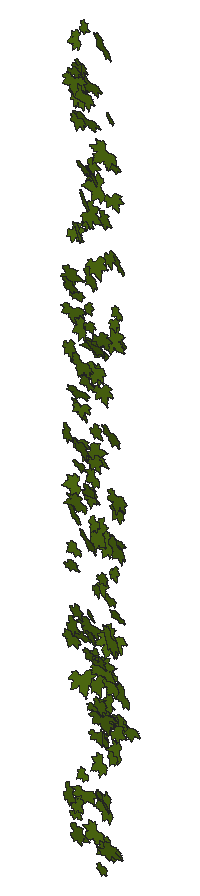
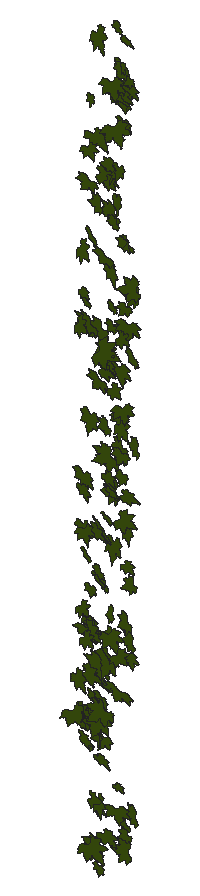
# SketchUp Ruby script. Lengths in inches.
U = 1.inch
M = Sketchup.active_model
def pt(a) = Geom::Point3d.new(a.map { |v| v * U })
def face(e, loops, mat)
  f = e.add_face(loops[0].map { |a| pt(a) })
  loops[1..].each { |l| e.add_face(l.map { |a| pt(a) }).erase! }
  f.material = f.back_material = mat if mat
  f
end
# faces: each face lists its corners as indices into pts; further lists are holes
def faces(e, pts, list, mat = nil) = list.each { |f| face(e, (f[0].is_a?(Array) ? f : [f]).map { |l| l.map { |i| pts[i] } }, mat) }
# xy, xz, yz: faces in a plane at the given z, y or x. An outline is a flat list of corners, or four numbers for a rectangle; further outlines are holes
def ring(l) = l.size == 4 ? [[l[0], l[1]], [l[2], l[1]], [l[2], l[3]], [l[0], l[3]]] : l.each_slice(2).to_a
def flat(e, list, mat, &to3) = list.each { |f| face(e, (f[0].is_a?(Array) ? f : [f]).map { |l| ring(l).map { |u, v| to3.(u, v) } }, mat) }
def xy(e, z, list, mat = nil) = flat(e, list, mat) { |x, y| [x, y, z] }
def xz(e, y, list, mat = nil) = flat(e, list, mat) { |x, z| [x, y, z] }
def yz(e, x, list, mat = nil) = flat(e, list, mat) { |y, z| [x, y, z] }
def lines(e, pts, list) = list.each { |a, b| e.add_line(pt(pts[a]), pt(pts[b])) }
# prism: a flat outline (further loops are holes) pulled along v
def prism(e, loops, v, mat = nil)
  f = face(e, loops, mat); d = Geom::Vector3d.new(v.map { |x| x * U })
  f.pushpull(f.normal.samedirection?(d) ? d.length : -d.length)
end
def box(e, o, s, mat = nil) = prism(e, [[o, [o[0] + s[0], o[1], o[2]], [o[0] + s[0], o[1] + s[1], o[2]], [o[0], o[1] + s[1], o[2]]]], [0, 0, s[2]], mat)
def at(x, y, z, deg = 0) = Geom::Transformation.translation(pt([x, y, z])) * Geom::Transformation.rotation(ORIGIN, Z_AXIS, deg.degrees)
def axes(o, x, y, z) = Geom::Transformation.new([*x, 0, *y, 0, *z, 0, *pt(o).to_a, 1])
def part(name) = M.definitions.add(name)
# library, detail: a bought-in or finely detailed component or shape, given as its bounding box
def library(name, o, s) = part(name).tap { |d| box(d.entities, o, s) }
def detail(e, o, s) = box(e.add_group.entities, o, s)
def put(e, d, t, mat = nil) = e.add_instance(d, t).tap { |i| i.material = mat if mat }
def group(e, t, mat = nil) = e.add_group.tap { |g| g.transformation = t; g.material = mat if mat }.entities
root = M.entities
M.materials.add("[Vegetation Blur 03]").color = [83, 114, 18]
c1 = part("ivy")
xy(c1.entities,0,[[0.782,0,0.786,0,0.787,0.005,0.789,0.009,0.821,0.072,0.875,0.147,1.001,0.272,1.073,0.331,1.137,0.363,1.178,0.379,1.223,0.384,1.272,0.383,1.311,0.374,1.36,0.355,1.399,0.334,1.491,0.285,1.541,0.244,1.583,0.199,1.617,0.15,1.64,0.128,1.662,0.115,1.717,0.105,1.745,0.093,1.784,0.054,1.819,0.057,1.854,0.064,1.882,0.075,1.896,0.074,1.91,0.071,1.937,0.063,1.964,0.053,1.99,0.038,2.016,0.015,2.034,0.002,2.04,0,2.038,0.003,2.036,0.007,2.033,0.038,2.036,0.068,2.045,0.1,2.055,0.116,2.064,0.123,2.077,0.129,2.088,0.129,2.106,0.132,2.118,0.13,2.179,0.132,2.207,0.133,2.225,0.133,2.242,0.138,2.22,0.162,2.207,0.186,2.206,0.213,2.212,0.236,2.228,0.262,2.247,0.274,2.298,0.283,2.355,0.294,2.37,0.296,2.376,0.295,2.377,0.3,2.377,0.303,2.385,0.329,2.411,0.37,2.426,0.392,2.449,0.407,2.511,0.426,2.561,0.444,2.619,0.466,2.589,0.469,2.561,0.476,2.501,0.5,2.449,0.516,2.424,0.523,2.401,0.535,2.377,0.556,2.372,0.568,2.36,0.575,2.268,0.586,2.225,0.592,2.207,0.599,2.194,0.61,2.143,0.65,2.13,0.664,2.122,0.682,2.123,0.7,2.13,0.719,2.148,0.75,2.17,0.781,2.195,0.807,2.221,0.828,2.284,0.874,2.291,0.88,2.288,0.887,2.276,0.9,2.267,0.916,2.265,0.933,2.273,0.967,2.292,1.002,2.313,1.03,2.334,1.054,2.348,1.067,2.358,1.074,2.363,1.076,2.362,1.081,2.35,1.094,2.347,1.11,2.35,1.143,2.359,1.18,2.385,1.254,2.415,1.324,2.448,1.393,2.45,1.4,2.446,1.398,2.44,1.394,2.427,1.383,2.402,1.36,2.376,1.339,2.345,1.324,2.305,1.309,2.282,1.303,2.273,1.306,2.245,1.294,2.212,1.287,2.187,1.291,2.163,1.301,2.142,1.316,2.134,1.327,2.124,1.325,2.09,1.292,2.053,1.259,2.014,1.234,1.973,1.215,1.954,1.21,1.931,1.208,1.909,1.212,1.893,1.22,1.879,1.233,1.872,1.248,1.867,1.281,1.864,1.319,1.821,1.258,1.773,1.197,1.726,1.141,1.698,1.121,1.679,1.116,1.666,1.117,1.647,1.122,1.632,1.129,1.62,1.141,1.617,1.154,1.617,1.219,1.621,1.254,1.623,1.268,1.623,1.281,1.618,1.314,1.606,1.346,1.603,1.375,1.607,1.403,1.603,1.467,1.599,1.499,1.605,1.525,1.614,1.552,1.629,1.577,1.635,1.589,1.629,1.587,1.618,1.582,1.596,1.566,1.581,1.556,1.568,1.552,1.557,1.55,1.545,1.553,1.531,1.562,1.522,1.572,1.504,1.591,1.486,1.611,1.474,1.631,1.457,1.666,1.455,1.684,1.457,1.698,1.452,1.715,1.444,1.728,1.424,1.754,1.419,1.772,1.423,1.786,1.434,1.819,1.444,1.848,1.446,1.855,1.44,1.861,1.43,1.867,1.386,1.904,1.349,1.948,1.326,1.973,1.31,1.995,1.288,2.048,1.284,2.153,1.287,2.254,1.284,2.255,1.282,2.253,1.278,2.247,1.274,2.237,1.266,2.216,1.226,2.125,1.208,2.076,1.184,2.033,1.155,1.984,1.135,1.942,1.111,1.899,1.083,1.861,1.053,1.85,1.059,1.83,1.061,1.809,1.056,1.79,1.049,1.767,1.04,1.749,1.018,1.733,0.994,1.726,0.942,1.734,0.95,1.6875,0.944,1.645,0.932,1.608,0.911,1.585,0.881,1.58,0.854,1.582,0.828,1.588,0.785,1.618,0.773,1.625,0.775,1.614,0.779,1.598,0.796,1.502,0.818,1.402,0.861,1.283,0.882,1.224,0.894,1.174,0.892,1.148,0.886,1.123,0.881,1.107,0.872,1.099,0.849,1.094,0.818,1.092,0.789,1.098,0.762,1.107,0.753,1.113,0.721,1.139,0.698,1.163,0.678,1.194,0.665,1.224,0.628,1.28,0.612,1.312,0.606,1.327,0.606,1.314,0.599,1.282,0.594,1.267,0.581,1.256,0.544,1.245,0.512,1.244,0.473,1.249,0.444,1.256,0.382,1.288,0.339,1.306,0.324,1.316,0.317,1.324,0.309,1.326,0.27,1.314,0.227,1.313,0.185,1.3125,0.152,1.317,0.122,1.328,0.092,1.345,0.073,1.353,0.079,1.338,0.092,1.308,0.117,1.249,0.13,1.215,0.139,1.164,0.147,1.148,0.157,1.136,0.163,1.122,0.174,1.086,0.177,1.067,0.182,1.054,0.186,1.043,0.191,1.038,0.211,1.028,0.237,1.005,0.25,0.974,0.253,0.96,0.25,0.944,0.242,0.914,0.243,0.906,0.249,0.902,0.26,0.894,0.289,0.88,0.307,0.873,0.322,0.862,0.364,0.799,0.403,0.738,0.431,0.709,0.439,0.691,0.441,0.678,0.4375,0.66,0.428,0.645,0.394,0.623,0.303,0.594,0.255,0.581,0.214,0.577,0.179,0.573,0.173,0.568,0.175,0.561,0.167,0.55,0.141,0.523,0.113,0.503,0.077,0.49,0.045,0.486,0.026,0.485,0.019,0.486,0.011,0.483,0,0.471,0.014,0.467,0.044,0.455,0.058,0.447,0.07,0.438,0.097,0.411,0.125,0.394,0.158,0.377,0.174,0.366,0.182,0.359,0.185,0.361,0.242,0.331,0.253,0.316,0.258,0.303,0.262,0.283,0.274,0.278,0.308,0.274,0.341,0.252,0.366,0.226,0.366,0.222,0.37,0.22,0.38,0.221,0.395,0.221,0.425,0.216,0.45,0.207,0.465,0.192,0.473,0.178,0.484,0.15,0.489,0.116,0.483,0.089,0.468,0.058,0.45,0.035,0.435,0.018,0.429,0.011,0.434,0.012,0.438,0.014,0.469,0.019,0.542,0.016,0.581,0.015,0.612,0.027,0.68,0.055,0.696,0.057,0.712,0.052,0.73,0.045,0.741,0.036,0.766,0.014]])
put(root,c1,axes([125.75,173.7,113.6875],[0.43906,-0.08807,-0.12908],[-0.15747,0.03053,-0.36003],[-0.0453,-0.95985,0.00039]),"[Vegetation Blur 03]")
put(root,c1,axes([125.56,173.7,123.65],[0.09017,-0.06413,0.35822],[0.42718,-0.20848,-0.07749],[-0.10559,-0.89821,-0.00759]),"[Vegetation Blur 03]")
put(root,c1,axes([125.48,173.7,130.61],[0.54749,0.01991,-0.01395],[-0.01748,0.04635,-0.4465],[0.00896,-1.12621,-0.01862]),"[Vegetation Blur 03]")
put(root,c1,axes([126.51,173.7,120.92],[0.16632,0.09986,-0.39596],[-0.48659,-0.03313,-0.13745],[0.03103,-1.05488,-0.03317]),"[Vegetation Blur 03]")
put(root,c1,axes([126.19,173.7,118.375],[0.23314,-0.02071,-0.23083],[-0.28282,0.0106,-0.19042],[-0.01038,-0.7542,0.00366]),"[Vegetation Blur 03]")
put(root,c1,axes([126.01,173.7,120.26],[0.37136,-0.15214,-0.22354],[-0.25515,0.22677,-0.30661],[-0.12403,-0.92207,-0.03852]),"[Vegetation Blur 03]")
put(root,c1,axes([126.41,173.7,125.78],[0.25339,0.01902,-0.3994],[-0.47391,0.29322,-0.19806],[-0.12245,-1.09547,-0.05995]),"[Vegetation Blur 03]")
put(root,c1,axes([125.61,173.7,116.9],[0.22705,-0.08947,0.23456],[0.29067,0.06726,-0.18337],[-0.00101,-0.75069,-0.04439]),"[Vegetation Blur 03]")
put(root,c1,axes([125.92,173.7,126.45],[0.41502,0.09791,-0.15811],[-0.19925,0.15826,-0.33295],[0.0098,-0.92912,-0.07337]),"[Vegetation Blur 03]")
put(root,c1,axes([126.49,173.7,121.94],[0.1638,-0.10041,-0.33523],[-0.41333,-0.07495,-0.13099],[0.01603,-0.90688,0.04794]),"[Vegetation Blur 03]")
put(root,c1,axes([125.47,173.7,131.78],[0.15315,-0.11376,0.42127],[0.51825,0.09795,-0.12133],[0.03021,-1.10363,-0.05419]),"[Vegetation Blur 03]")
put(root,c1,axes([126.45,173.7,135.02],[0.17953,-0.09504,-0.30608],[-0.36446,0.18198,-0.15128],[-0.09974,-0.83603,0.00186]),"[Vegetation Blur 03]")
put(root,c1,axes([126.57,173.7,130.08],[0.09179,0.09251,-0.29251],[-0.35994,0.08732,-0.07089],[-0.03033,-0.7563,-0.04396]),"[Vegetation Blur 03]")
put(root,c1,axes([125.61,173.7,104.72],[0.09186,-0.01547,0.40746],[0.48625,-0.23456,-0.07442],[-0.11344,-1.01793,0.01096]),"[Vegetation Blur 03]")
put(root,c1,axes([125.66,173.7,131.4],[0.10455,-0.16948,0.36645],[0.45413,-0.0579,-0.09052],[-0.04648,-0.94693,-0.06005]),"[Vegetation Blur 03]")
put(root,c1,axes([125.55,173.7,128.5],[0.35673,-0.12377,0.22075],[0.25958,-0.16822,-0.29423],[-0.09696,-0.90576,0.02448]),"[Vegetation Blur 03]")
put(root,c1,axes([125.58,173.7,142.68],[0.55862,-0.01173,0.01902],[0.02312,-0.03492,-0.45573],[-0.0064,-1.15001,0.01364]),"[Vegetation Blur 03]")
put(root,c1,axes([125.77,173.7,142.86],[0.27413,-0.06194,0.16545],[0.20434,0.02916,-0.2238],[-0.01572,-0.70099,-0.02393]),"[Vegetation Blur 03]")
put(root,c1,axes([126.52,173.7,113.8],[0.1902,0.17643,-0.26649],[-0.33646,0.03567,-0.15623],[0.02775,-0.7768,-0.0677]),"[Vegetation Blur 03]")
put(root,c1,axes([125.88,173.7,131.2],[0.28384,0.00263,0.11756],[0.14245,0.09199,-0.22943],[0.02136,-0.64851,-0.03207]),"[Vegetation Blur 03]")
put(root,c1,axes([125.78,173.7,113.66],[0.12722,-0.05638,0.35512],[0.42991,-0.13892,-0.10606],[-0.07252,-0.92248,-0.00573]),"[Vegetation Blur 03]")
put(root,c1,axes([126.54,173.7,145.1875],[0.2034,-0.19719,-0.25526],[-0.32297,-0.00076,-0.17132],[-0.05192,-0.76775,0.06573]),"[Vegetation Blur 03]")
put(root,c1,axes([125.72,173.7,134.24],[0.23996,0.10055,0.29847],[0.36879,-0.09254,-0.19259],[-0.01117,-0.89532,0.05342]),"[Vegetation Blur 03]")
put(root,c1,axes([125.92,173.7,104.02],[0.1988,-0.0106,0.20658],[0.25313,-0.00387,-0.16228],[-0.00466,-0.6623,-0.00236]),"[Vegetation Blur 03]")
put(root,c1,axes([126.29,173.7,140.93],[0.48948,0.16058,-0.27855],[-0.34964,0.16113,-0.39462],[0.01829,-1.21733,-0.08898]),"[Vegetation Blur 03]")
put(root,c1,axes([126.07,173.7,140.77],[0.4277,-0.13208,-0.01923],[-0.02433,-0.00684,-0.35292],[-0.0639,-0.88143,0.00562]),"[Vegetation Blur 03]")
put(root,c1,axes([126.15,173.7,122.61],[0.33381,-0.09287,0.01816],[0.028,0.08748,-0.27236],[-0.04181,-0.68286,-0.03736]),"[Vegetation Blur 03]")
put(root,c1,axes([126,173.7,104.45],[0.18478,0.02807,0.2907],[0.35178,-0.14758,-0.1467],[-0.05752,-0.81244,0.03669]),"[Vegetation Blur 03]")
put(root,c1,axes([126.02,173.7,123.66],[0.39754,-0.01789,0.09307],[0.11433,0.03939,-0.32408],[-0.00307,-0.85015,-0.01697]),"[Vegetation Blur 03]")
put(root,c1,axes([125.92,173.7,114.79],[0.32691,-0.16543,0.24576],[0.30294,-0.04245,-0.2729],[-0.07327,-0.91364,-0.03182]),"[Vegetation Blur 03]")
put(root,c1,axes([126.15,173.7,125.57],[0.37993,0.04432,0.03279],[0.04106,-0.03097,-0.31026],[0.01982,-0.78558,0.01408]),"[Vegetation Blur 03]")
put(root,c1,axes([126.0625,173.7,143.3125],[0.38821,-0.11193,0.10755],[0.13579,0.05066,-0.31818],[-0.04343,-0.84212,-0.03344]),"[Vegetation Blur 03]")
put(root,c1,axes([126.22,173.7,142.46],[0.60025,-0.11632,-0.20653],[-0.25299,0.02521,-0.49198],[-0.05685,-1.34025,0.00867]),"[Vegetation Blur 03]")
put(root,c1,axes([126.16,173.7,128.3],[0.58763,-0.14391,-0.14762],[-0.17735,0.08172,-0.48275],[-0.07846,-1.26257,-0.01442]),"[Vegetation Blur 03]")
put(root,c1,axes([126.74,173.7,130.34],[0.30417,-0.25351,-0.27604],[-0.3464,0.04167,-0.26026],[-0.0979,-0.93513,0.06323]),"[Vegetation Blur 03]")
put(root,c1,axes([125.97,173.7,141.55],[0.34233,0.0367,0.25351],[0.30852,-0.16299,-0.27378],[-0.04025,-0.93715,0.05755]),"[Vegetation Blur 03]")
put(root,c1,axes([126.19,173.7,105.64],[0.52025,0.05923,-0.06815],[-0.08303,-0.02209,-0.42521],[0.03012,-1.08405,0.00494]),"[Vegetation Blur 03]")
put(root,c1,axes([126.03,173.7,102.73],[0.10484,-0.11239,0.45286],[0.55605,-0.06423,-0.08825],[-0.04094,-1.16025,-0.03898]),"[Vegetation Blur 03]")
put(root,c1,axes([126.28,173.7,143.62],[0.38177,-0.16884,0.00908],[0.01686,0.05275,-0.31784],[-0.08106,-0.78418,-0.02334]),"[Vegetation Blur 03]")
put(root,c1,axes([126.36,173.7,138.35],[0.38893,-0.1332,-0.05202],[-0.05011,0.16639,-0.31658],[-0.07577,-0.79377,-0.05763]),"[Vegetation Blur 03]")
put(root,c1,axes([126.95,173.7,127.25],[0.18993,0.03098,-0.27697],[-0.33885,0.07408,-0.15347],[-0.02412,-0.79685,-0.02503]),"[Vegetation Blur 03]")
put(root,c1,axes([126.75,173.7,106.74],[0.21979,-0.07452,-0.15702],[-0.1954,-0.04663,-0.1787],[-0.01213,-0.59927,0.03343]),"[Vegetation Blur 03]")
put(root,c1,axes([126.62,173.7,136.88],[0.36908,-0.2283,-0.18774],[-0.2052,0.23015,-0.31272],[-0.15204,-0.86483,-0.03366]),"[Vegetation Blur 03]")
put(root,c1,axes([126.53,173.7,142.97],[0.53586,0.00327,-0.21137],[-0.25728,0.14717,-0.4341],[-0.0297,-1.21585,-0.05311]),"[Vegetation Blur 03]")
put(root,c1,axes([126.54,173.7,145.14],[0.05613,0.01305,0.23736],[0.28926,-0.0672,-0.04498],[-0.03088,-0.6058,0.0101]),"[Vegetation Blur 03]")
put(root,c1,axes([125.87,173.7,111.34],[0.58242,0.07305,0.2372],[0.29248,-0.20649,-0.46835],[-0.01349,-1.32342,0.08617]),"[Vegetation Blur 03]")
put(root,c1,axes([126.73,173.7,114.7],[0.47827,0.03325,-0.27343],[-0.33498,0.10885,-0.38819],[-0.01718,-1.19669,-0.04291]),"[Vegetation Blur 03]")
put(root,c1,axes([126.07,173.7,123.72],[0.52923,-0.27231,0.14829],[0.19148,0.04522,-0.44212],[-0.11773,-1.15056,-0.05247]),"[Vegetation Blur 03]")
put(root,c1,axes([127.27,173.7,137.81],[0.1507,0.00007,-0.27274],[-0.3307,0.10871,-0.1217],[-0.04814,-0.74651,-0.01775]),"[Vegetation Blur 03]")
put(root,c1,axes([126.54,173.7,119.22],[0.58057,-0.26082,-0.16045],[-0.16911,0.27993,-0.47915],[-0.16161,-1.22989,-0.07503]),"[Vegetation Blur 03]")
put(root,c1,axes([127.72,173.7,129.36],[0.08849,0.22325,-0.50781],[-0.6312,-0.01504,-0.0743],[0.02262,-1.29319,-0.0868]),"[Vegetation Blur 03]")
put(root,c1,axes([126.65,173.7,135.03],[0.11812,0.02268,0.27727],[0.33763,-0.09352,-0.0946],[-0.03936,-0.73423,0.02061]),"[Vegetation Blur 03]")
put(root,c1,axes([126.99,173.7,133.14],[0.45147,-0.25025,-0.22719],[-0.26949,0.14362,-0.38159],[-0.1402,-1.08195,0.00189]),"[Vegetation Blur 03]")
put(root,c1,axes([126.75,173.7,129.9],[0.26219,-0.05379,0.13773],[0.16863,-0.0189,-0.21498],[-0.02696,-0.64136,-0.00522]),"[Vegetation Blur 03]")
put(root,c1,axes([126.92,173.7,138.26],[0.41315,-0.18544,-0.14251],[-0.1576,0.18691,-0.3426],[-0.11735,-0.90388,-0.04161]),"[Vegetation Blur 03]")
put(root,c1,axes([126.79,173.7,130.78],[0.19571,-0.04059,0.18321],[0.21938,-0.10557,-0.15978],[-0.05153,-0.6037,0.01562]),"[Vegetation Blur 03]")
put(root,c1,axes([127.29,173.7,122.61],[0.30292,-0.11557,-0.26319],[-0.32214,0.05514,-0.25077],[-0.05807,-0.90879,0.01825]),"[Vegetation Blur 03]")
put(root,c1,axes([126.88,173.7,121.49],[0.2893,-0.06946,0.05279],[0.06075,-0.07196,-0.23668],[-0.04039,-0.60575,0.02206]),"[Vegetation Blur 03]")
put(root,c1,axes([126.92,173.7,137.93],[0.04916,0.02287,0.27993],[0.3427,0.03405,-0.04052],[0.01796,-0.71221,0.00705]),"[Vegetation Blur 03]")
put(root,c1,axes([126.87,173.7,129.14],[0.46406,-0.05319,-0.06714],[-0.07481,0.21257,-0.37089],[-0.04289,-0.94624,-0.07954]),"[Vegetation Blur 03]")
put(root,c1,axes([127.86,173.7,128.08],[0.07216,-0.07343,-0.39325],[-0.48158,0.07012,-0.06092],[-0.03906,-1.00014,0.0246]),"[Vegetation Blur 03]")
put(root,c1,axes([127.3,173.7,104.21],[0.3982,-0.07833,-0.27853],[-0.34327,-0.06231,-0.32413],[-0.0091,-1.07738,0.039]),"[Vegetation Blur 03]")
put(root,c1,axes([126.58,173.7,135.25],[0.15618,0.05581,0.47785],[0.58342,-0.13447,-0.12454],[-0.05625,-1.2397,0.03502]),"[Vegetation Blur 03]")
put(root,c1,axes([127.91,173.7,138.125],[0.18243,-0.13935,-0.48722],[-0.59996,0.02639,-0.15082],[-0.03212,-1.28429,0.04976]),"[Vegetation Blur 03]")
put(root,c1,axes([126.79,173.7,121.33],[0.43109,-0.16307,0.09857],[0.11374,-0.09903,-0.3571],[-0.08905,-0.91592,0.02106]),"[Vegetation Blur 03]")
put(root,c1,axes([126.875,173.7,113.92],[0.34195,-0.22556,0.12659],[0.16367,0.01646,-0.28987],[-0.09636,-0.7725,-0.04314]),"[Vegetation Blur 03]")
put(root,c1,axes([127.03,173.7,114.86],[0.1642,-0.18374,0.20113],[0.24769,-0.08699,-0.14719],[-0.08574,-0.60314,-0.04004]),"[Vegetation Blur 03]")
put(root,c1,axes([126.66,173.7,113.01],[0.64437,-0.16461,0.01325],[0.02704,0.17964,-0.52482],[-0.07702,-1.31419,-0.0734]),"[Vegetation Blur 03]")
put(root,c1,axes([126.71,173.7,120.94],[0.20255,-0.18759,0.41357],[0.50926,-0.09194,-0.17269],[-0.07578,-1.11921,-0.05513]),"[Vegetation Blur 03]")
put(root,c1,axes([126.51,173.7,122.86],[0.3615,0.01419,0.44771],[0.54841,0.02846,-0.29509],[0.01534,-1.35164,-0.00151]),"[Vegetation Blur 03]")
put(root,c1,axes([127.65,173.7,145.39],[0.37946,-0.0754,-0.40939],[-0.47883,0.34147,-0.30552],[-0.15388,-1.24846,-0.05884]),"[Vegetation Blur 03]")
put(root,c1,axes([127.28,173.7,120.12],[0.34373,-0.18323,-0.04475],[-0.06771,-0.09451,-0.28552],[-0.07969,-0.71,0.04955]),"[Vegetation Blur 03]")
put(root,c1,axes([127.15,173.7,112.84],[0.19414,-0.08015,0.20136],[0.24242,-0.09451,-0.1616],[-0.0602,-0.6391,-0.00136]),"[Vegetation Blur 03]")
put(root,c1,axes([127.01,173.7,128.1],[0.54066,-0.11979,-0.01485],[-0.02304,-0.09186,-0.44216],[-0.05647,-1.10941,0.03821]),"[Vegetation Blur 03]")
put(root,c1,axes([126.99,173.7,122.84],[0.30004,-0.03578,0.23182],[0.28092,-0.09842,-0.24458],[-0.04545,-0.84451,0.01868]),"[Vegetation Blur 03]")
put(root,c1,axes([127.03,173.7,108.78],[0.44477,-0.01678,0.0841],[0.10333,0.04659,-0.36253],[-0.00282,-0.93833,-0.0195]),"[Vegetation Blur 03]")
put(root,c1,axes([127.1,173.7,124.4375],[0.23733,-0.08095,0.26556],[0.32364,-0.07275,-0.19614],[-0.05179,-0.82556,-0.00876]),"[Vegetation Blur 03]")
put(root,c1,axes([126.89,173.7,133.21],[0.44354,0.00148,0.25414],[0.30752,-0.17731,-0.35733],[-0.04893,-1.101,0.05789]),"[Vegetation Blur 03]")
put(root,c1,axes([127.64,173.7,105.88],[0.41747,-0.18159,-0.28175],[-0.32214,0.27535,-0.34584],[-0.15229,-1.08022,-0.04079]),"[Vegetation Blur 03]")
put(root,c1,axes([127.3125,173.7,116.32],[0.21446,-0.11197,0.17329],[0.20462,-0.11686,-0.18055],[-0.07858,-0.60992,0.00278]),"[Vegetation Blur 03]")
put(root,c1,axes([126.8,173.7,109.94],[0.46309,-0.00814,0.32802],[0.3991,0.15897,-0.37467],[0.04767,-1.25175,-0.04972]),"[Vegetation Blur 03]")
put(root,c1,axes([127.05,173.7,111.31],[0.35031,-0.0224,0.27157],[0.32357,-0.21117,-0.28075],[-0.0784,-0.97156,0.05476]),"[Vegetation Blur 03]")
put(root,c1,axes([127.76,173.7,107.9],[0.35443,-0.19304,-0.2419],[-0.30587,-0.0509,-0.29211],[-0.05567,-0.94941,0.06485]),"[Vegetation Blur 03]")
put(root,c1,axes([127.72,173.7,139.99],[0.532,-0.08529,-0.32199],[-0.3962,-0.04622,-0.4341],[-0.01987,-1.36215,0.03489]),"[Vegetation Blur 03]")
put(root,c1,axes([127.07,173.7,118.68],[0.16553,0.17765,0.51158],[0.60894,-0.40708,-0.109],[-0.17196,-1.2705,0.10646]),"[Vegetation Blur 03]")
put(root,c1,axes([127.84,173.7,109.0625],[0.30175,-0.15566,-0.18852],[-0.22184,0.13329,-0.25383],[-0.09933,-0.77056,-0.00582]),"[Vegetation Blur 03]")
put(root,c1,axes([128.33,173.7,105.9],[0.23881,-0.20013,-0.4704],[-0.57401,0.16163,-0.20491],[-0.11037,-1.27363,0.04791]),"[Vegetation Blur 03]")
put(root,c1,axes([127.59,173.7,102.07],[0.31854,-0.11206,-0.01065],[-0.01233,0.01101,-0.26373],[-0.05462,-0.65595,-0.00261]),"[Vegetation Blur 03]")
put(root,c1,axes([127.03,173.7,109.81],[0.67064,-0.03297,0.06761],[0.08405,0.14038,-0.54453],[-0.00745,-1.38343,-0.05687]),"[Vegetation Blur 03]")
put(root,c1,axes([127.37,173.7,110.65],[0.43055,-0.17357,0.04955],[0.0586,-0.03425,-0.35804],[-0.08583,-0.8941,0.0041]),"[Vegetation Blur 03]")
put(root,c1,axes([127.95,173.7,103.68],[0.46314,0.05825,-0.39602],[-0.48604,0.04033,-0.37767],[0.00535,-1.37976,-0.02776]),"[Vegetation Blur 03]")
put(root,c1,axes([127.51,173.7,116.93],[0.24085,-0.07286,0.19486],[0.23769,-0.04913,-0.19858],[-0.04198,-0.69616,-0.00638]),"[Vegetation Blur 03]")
put(root,c1,axes([128.24,173.7,119.6875],[0.31165,-0.23246,-0.38206],[-0.4746,0.04633,-0.26229],[-0.08166,-1.15634,0.0663]),"[Vegetation Blur 03]")
put(root,c1,axes([127.19,173.7,129.35],[0.40049,-0.10291,0.28569],[0.35224,0.02026,-0.32774],[-0.03114,-1.09438,-0.03293]),"[Vegetation Blur 03]")
put(root,c1,axes([128.46,173.7,114.65],[0.20411,-0.06117,-0.44075],[-0.53473,0.15542,-0.16833],[-0.08116,-1.17781,0.00068]),"[Vegetation Blur 03]")
put(root,c1,axes([127.49,173.7,116.47],[0.2517,0.01272,0.24338],[0.28699,-0.2291,-0.19581],[-0.08127,-0.76965,0.06231]),"[Vegetation Blur 03]")
put(root,c1,axes([127.28,173.7,126.8],[0.46612,-0.06322,0.21313],[0.25778,-0.10592,-0.38046],[-0.05188,-1.09436,0.02451]),"[Vegetation Blur 03]")
put(root,c1,axes([127.07,173.7,111.9375],[0.4004,-0.01607,0.44585],[0.54595,-0.04146,-0.32681],[-0.02086,-1.39316,0.00458]),"[Vegetation Blur 03]")
put(root,c1,axes([128.54,173.7,111.05],[0.07522,-0.13511,-0.31021],[-0.37954,0.11629,-0.06927],[-0.06884,-0.78881,0.04292]),"[Vegetation Blur 03]")
put(root,c1,axes([128.7,173.7,112.33],[0.13923,-0.07198,-0.4584],[-0.56199,0.04465,-0.11479],[-0.02951,-1.18996,0.02342]),"[Vegetation Blur 03]")
put(root,c1,axes([128.11,173.7,139.09],[0.32097,0.04197,-0.19874],[-0.24426,0.07998,-0.2601],[-0.00735,-0.82521,-0.03532]),"[Vegetation Blur 03]")
put(root,c1,axes([127.63,173.7,135.48],[0.11949,-0.05949,0.35767],[0.43416,-0.12523,-0.09989],[-0.06637,-0.92633,-0.00946]),"[Vegetation Blur 03]")
put(root,c1,axes([128.5,173.7,114.05],[0.16976,0.07158,-0.29867],[-0.3654,0.12339,-0.13369],[-0.04012,-0.82092,-0.04613]),"[Vegetation Blur 03]")
put(root,c1,axes([128.14,173.7,141.46],[0.26677,-0.13263,-0.08131],[-0.08808,0.11667,-0.22242],[-0.07951,-0.57427,-0.02641]),"[Vegetation Blur 03]")
put(root,c1,axes([128.02,173.7,116.28],[0.33233,-0.0945,-0.02615],[-0.02986,0.03657,-0.27359],[-0.04737,-0.68607,-0.01098]),"[Vegetation Blur 03]")
put(root,c1,axes([128.74,173.7,134.07],[0.15729,0.04975,-0.38701],[-0.46067,0.26502,-0.11935],[-0.11503,-0.99334,-0.05122]),"[Vegetation Blur 03]")
put(root,c1,axes([128.05,173.7,114.71],[0.56265,-0.26157,-0.25412],[-0.30853,0.09554,-0.47049],[-0.13384,-1.31983,0.01631]),"[Vegetation Blur 03]")
put(root,c1,axes([128.25,173.7,119.48],[0.35115,0.05857,-0.18722],[-0.23024,0.1649,-0.27952],[-0.02054,-0.84722,-0.06735]),"[Vegetation Blur 03]")
put(root,c1,axes([127.61,173.7,102.55],[0.26007,-0.08689,0.38147],[0.46915,0.07766,-0.21026],[0.0126,-1.09796,-0.04506]),"[Vegetation Blur 03]")
put(root,c1,axes([127.72,173.7,114.27],[0.61939,0.05734,-0.0417],[-0.04546,-0.22498,-0.49845],[0.03634,-1.25897,0.08717]),"[Vegetation Blur 03]")
put(root,c1,axes([127.86,173.7,113.87],[0.12985,0.03067,0.35023],[0.42444,-0.14892,-0.10276],[-0.06505,-0.91052,0.02861]),"[Vegetation Blur 03]")
put(root,c1,axes([128.66,173.7,115.54],[0.17674,0.08976,-0.26223],[-0.3229,0.11764,-0.13863],[-0.02967,-0.7454,-0.05345]),"[Vegetation Blur 03]")
put(root,c1,axes([127.85,173.7,125.13],[0.58072,-0.2362,-0.06513],[-0.0644,0.17074,-0.47989],[-0.12408,-1.1941,-0.05574]),"[Vegetation Blur 03]")
put(root,c1,axes([128.9375,173.7,130.0625],[0.08767,0.08949,-0.34433],[-0.41588,0.19217,-0.06267],[-0.08326,-0.86566,-0.04951]),"[Vegetation Blur 03]")
put(root,c1,axes([128.58,173.7,114.08],[0.25432,-0.19046,-0.24423],[-0.28944,0.16036,-0.22043],[-0.11975,-0.79207,0.0141]),"[Vegetation Blur 03]")
put(root,c1,axes([127.82,173.7,136.9],[0.40459,0.02303,0.19859],[0.2435,-0.01333,-0.3302],[0.00625,-0.97145,0.00924]),"[Vegetation Blur 03]")
put(root,c1,axes([127.96,173.7,133.91],[0.28926,-0.09005,0.2261],[0.2622,-0.20395,-0.23621],[-0.09958,-0.79857,0.03483]),"[Vegetation Blur 03]")
put(root,c1,axes([129.01,173.7,108.75],[0.10121,-0.15146,-0.36108],[-0.44341,0.10659,-0.08981],[-0.06746,-0.92784,0.04863]),"[Vegetation Blur 03]")
put(root,c1,axes([128.34,173.7,108.16],[0.30014,-0.14068,-0.03498],[-0.05049,-0.06238,-0.24906],[-0.06295,-0.62077,0.03295]),"[Vegetation Blur 03]")
put(root,c1,axes([128.72,173.7,131.5],[0.20022,-0.05357,-0.19807],[-0.24233,0.03356,-0.1646],[-0.02917,-0.64656,0.00787]),"[Vegetation Blur 03]")
put(root,c1,axes([129.03,173.7,110.2],[0.11196,0.05174,-0.31654],[-0.38834,-0.01941,-0.09199],[0.01605,-0.83049,-0.01757]),"[Vegetation Blur 03]")
put(root,c1,axes([127.79,173.7,129.24],[0.28098,0.0713,0.44477],[0.5442,-0.14112,-0.22543],[-0.04527,-1.25382,0.05067]),"[Vegetation Blur 03]")
put(root,c1,axes([128.28,173.7,130.61],[0.25172,-0.04798,0.1294],[0.15152,-0.12662,-0.20371],[-0.0522,-0.59895,0.0327]),"[Vegetation Blur 03]")
put(root,c1,axes([128.38,173.7,119.53],[0.559,-0.25408,-0.226],[-0.26774,0.14716,-0.46713],[-0.14227,-1.27524,-0.00888]),"[Vegetation Blur 03]")
put(root,c1,axes([128.29,173.7,117.52],[0.23635,-0.06465,0.19523],[0.22776,-0.16748,-0.19239],[-0.07957,-0.67142,0.02919]),"[Vegetation Blur 03]")
put(root,c1,axes([128.5625,173.7,121.35],[0.41365,-0.19736,-0.16762],[-0.20533,0.04633,-0.34609],[-0.09602,-0.94924,0.01796]),"[Vegetation Blur 03]")
put(root,c1,axes([128.32,173.7,108.81],[0.09158,0.04301,0.34718],[0.42504,-0.06647,-0.07338],[-0.02723,-0.89296,0.02219]),"[Vegetation Blur 03]")
put(root,c1,axes([128.97,173.7,111.93],[0.35185,-0.14327,-0.37157],[-0.44566,0.19161,-0.29272],[-0.11623,-1.16844,-0.00244]),"[Vegetation Blur 03]")
put(root,c1,axes([128.22,173.7,121.91],[0.59559,-0.20487,-0.02237],[-0.02751,0.00349,-0.49282],[-0.09953,-1.2269,0.00233]),"[Vegetation Blur 03]")
put(root,c1,axes([128.83,173.7,110.13],[0.45581,0.11699,-0.31525],[-0.38742,-0.0162,-0.37405],[0.04848,-1.22937,-0.02507]),"[Vegetation Blur 03]")
